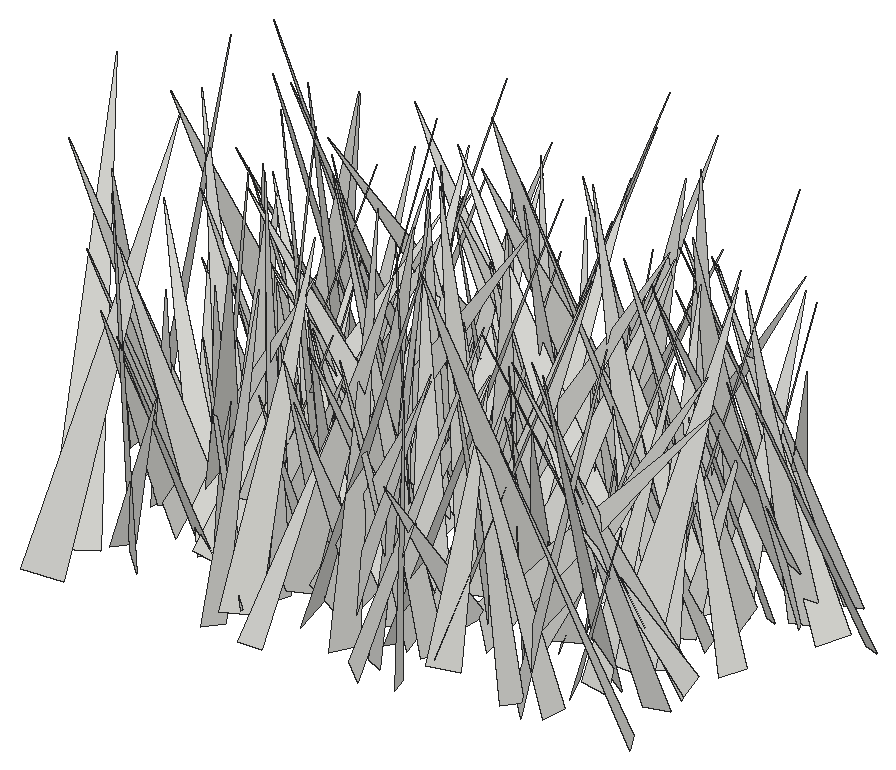
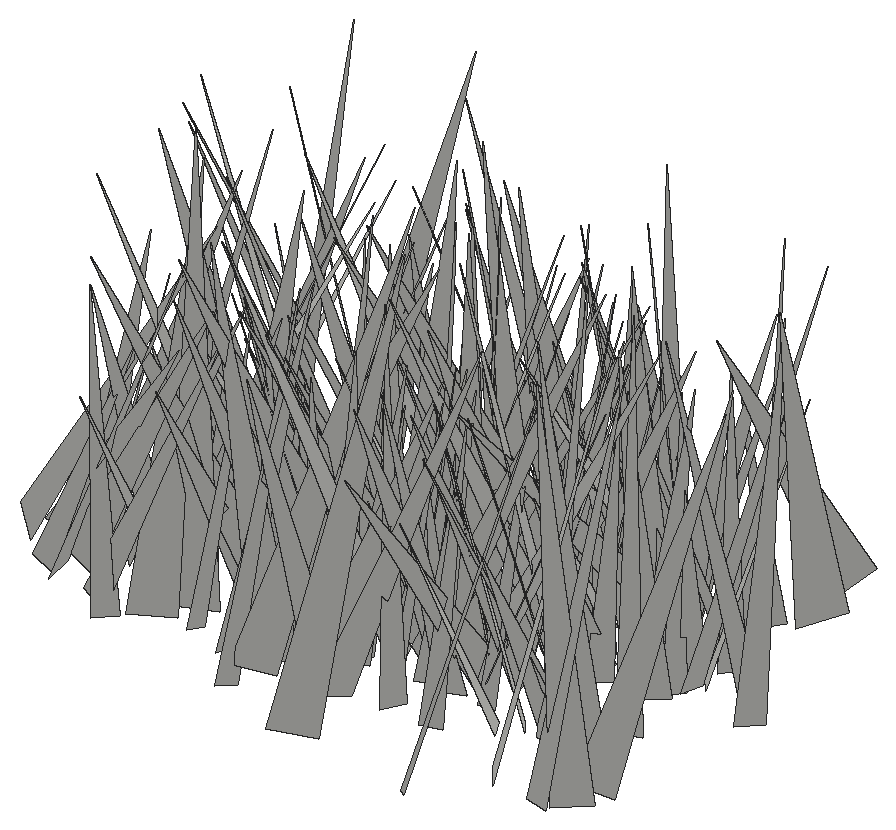
# SketchUp Ruby script. Lengths in inches.
U = 1.inch
M = Sketchup.active_model
def pt(a) = Geom::Point3d.new(a.map { |v| v * U })
def face(e, loops, mat)
  f = e.add_face(loops[0].map { |a| pt(a) })
  loops[1..].each { |l| e.add_face(l.map { |a| pt(a) }).erase! }
  f.material = f.back_material = mat if mat
  f
end
# faces: each face lists its corners as indices into pts; further lists are holes
def faces(e, pts, list, mat = nil) = list.each { |f| face(e, (f[0].is_a?(Array) ? f : [f]).map { |l| l.map { |i| pts[i] } }, mat) }
# xy, xz, yz: faces in a plane at the given z, y or x. An outline is a flat list of corners, or four numbers for a rectangle; further outlines are holes
def ring(l) = l.size == 4 ? [[l[0], l[1]], [l[2], l[1]], [l[2], l[3]], [l[0], l[3]]] : l.each_slice(2).to_a
def flat(e, list, mat, &to3) = list.each { |f| face(e, (f[0].is_a?(Array) ? f : [f]).map { |l| ring(l).map { |u, v| to3.(u, v) } }, mat) }
def xy(e, z, list, mat = nil) = flat(e, list, mat) { |x, y| [x, y, z] }
def xz(e, y, list, mat = nil) = flat(e, list, mat) { |x, z| [x, y, z] }
def yz(e, x, list, mat = nil) = flat(e, list, mat) { |y, z| [x, y, z] }
def lines(e, pts, list) = list.each { |a, b| e.add_line(pt(pts[a]), pt(pts[b])) }
# prism: a flat outline (further loops are holes) pulled along v
def prism(e, loops, v, mat = nil)
  f = face(e, loops, mat); d = Geom::Vector3d.new(v.map { |x| x * U })
  f.pushpull(f.normal.samedirection?(d) ? d.length : -d.length)
end
def box(e, o, s, mat = nil) = prism(e, [[o, [o[0] + s[0], o[1], o[2]], [o[0] + s[0], o[1] + s[1], o[2]], [o[0], o[1] + s[1], o[2]]]], [0, 0, s[2]], mat)
def at(x, y, z, deg = 0) = Geom::Transformation.translation(pt([x, y, z])) * Geom::Transformation.rotation(ORIGIN, Z_AXIS, deg.degrees)
def axes(o, x, y, z) = Geom::Transformation.new([*x, 0, *y, 0, *z, 0, *pt(o).to_a, 1])
def part(name) = M.definitions.add(name)
# library, detail: a bought-in or finely detailed component or shape, given as its bounding box
def library(name, o, s) = part(name).tap { |d| box(d.entities, o, s) }
def detail(e, o, s) = box(e.add_group.entities, o, s)
def put(e, d, t, mat = nil) = e.add_instance(d, t).tap { |i| i.material = mat if mat }
def group(e, t, mat = nil) = e.add_group.tap { |g| g.transformation = t; g.material = mat if mat }.entities
root = M.entities
c1 = part("fur_instance\#9")
p = [[0.8125,0,1.79],[0.67,-0.02,1.48],[0,-0.11,0],[0,0.11,0]]
faces(c1.entities,p,[[0,1,2,3]])
put(root,c1,axes([471.03,125.22,-21.86],[3.80015,2.05854,2.10545],[1.83657,-4.34391,0.93228],[-2.30164,-0.0674,4.22014]))
put(root,c1,axes([459.39,126.23,-21.86],[-4.34525,-4.69158,2.51984],[-5.05188,4.66036,-0.03462],[1.68493,1.87398,6.3946]))
put(root,c1,axes([458.42,126.88,-21.86],[3.1539,-2.32332,0.00557],[-2.32207,-3.15188,0.13648],[0.07647,0.11319,3.91488]))
put(root,c1,axes([479.16,126.97,-21.86],[-4.6266,-2.97065,0.07987],[-2.96143,4.59663,-0.58091],[-0.24706,0.53178,5.46742]))
put(root,c1,axes([465.68,124.31,-21.86],[-2.96386,2.60362,0.59977],[2.15648,2.85999,-1.75873],[1.5774,0.98217,3.53132]))
put(root,c1,axes([463.93,124.63,-21.86],[4.93577,0.48548,2.66433],[-0.37318,-5.36398,1.66873],[-2.68236,1.63958,4.67042]))
put(root,c1,axes([467.54,126.71,-21.66],[3.43659,4.37627,1.35344],[4.55407,-3.08156,-1.59944],[0.49399,-2.03617,5.32951]))
put(root,c1,axes([469.32,125.03,-21.86],[4.12664,4.96749,0.53315],[4.97839,-4.14664,0.10195],[-0.41933,-0.34468,6.45715]))
put(root,c1,axes([466.84,128.88,-21.86],[4.72297,-1.05883,1.70864],[-0.28791,-4.67444,-2.10088],[-1.98939,-1.83725,4.36049]))
put(root,c1,axes([464.3125,125.79,-21.66],[-4.28089,-1.18354,0.47624],[-1.27514,3.91753,-1.72642],[-0.03977,1.79046,4.09221]))
put(root,c1,axes([476.07,129.68,-21.66],[-2.59583,-7.17613,0.91864],[-6.91744,2.74775,1.9178],[2.11891,0.17907,7.38629]))
put(root,c1,axes([460.64,128.33,-21.86],[-1.93771,-4.14246,0.35212],[-4.15628,1.93921,-0.05843],[0.0961,0.34375,4.57288]))
put(root,c1,axes([465.97,127.15,-21.86],[7.81228,1.65656,1.00866],[1.73052,-7.84393,-0.52089],[-0.87571,-0.72239,7.96898]))
put(root,c1,axes([474.79,126.61,-21.86],[4.81614,4.80746,1.57054],[5.00941,-4.83285,-0.56818],[-0.69571,-1.51836,6.78115]))
put(root,c1,axes([469.63,127.7,-21.86],[-4.87581,-1.54153,0.97742],[-1.54685,4.96967,0.12147],[0.96896,0.17664,5.11224]))
put(root,c1,axes([465.83,127.86,-21.66],[0.54416,-5.67013,1.84078],[-5.27926,0.40028,2.79359],[2.76917,1.87733,4.9641]))
put(root,c1,axes([470.54,129.66,-21.66],[3.27584,-2.78093,0.2499],[-2.38988,-2.99185,-1.96583],[-1.44378,-1.35736,3.82103]))
put(root,c1,axes([464.33,125.4375,-21.66],[-4.85985,3.92503,1.53679],[3.59209,5.08366,-1.6245],[2.20555,0.36911,6.032]))
put(root,c1,axes([459.75,130.27,-21.86],[7.63705,-2.12328,0.08153],[-2.0044,-7.29978,-2.35267],[-0.70524,-2.24596,7.56953]))
put(root,c1,axes([468.42,125.72,-21.66],[-7.01527,0.64484,2.20419],[0.06996,7.14138,-1.86657],[2.29551,1.75305,6.79307]))
put(root,c1,axes([476.05,126.86,-21.86],[-6.46685,-0.99912,0.02995],[-0.985,6.33639,-1.3035],[-0.17003,1.29271,6.41243]))
put(root,c1,axes([471.46,126.95,-21.86],[-2.32023,4.26891,1.78267],[4.38145,2.66784,-0.68595],[1.48474,-1.20167,4.81004]))
put(root,c1,axes([457.87,123.47,-21.66],[-6.65412,4.03174,0.74119],[3.28122,6.08544,-3.64454],[2.45722,2.79179,6.87384]))
put(root,c1,axes([464.7,127.56,-21.66],[5.22316,-4.20753,1.34718],[-4.41725,-5.01042,1.47756],[-0.07792,1.998,6.54228]))
put(root,c1,axes([460.52,128.99,-21.66],[-5.0365,1.95588,2.0654],[2.56555,4.93734,1.5806],[1.22852,-2.29236,5.16658]))
put(root,c1,axes([469.27,129.31,-21.86],[-0.62326,-5.57048,0.69706],[-5.46922,0.44429,-1.33972],[-1.26641,0.82277,5.44278]))
put(root,c1,axes([475.54,128.57,-21.86],[4.06757,1.21437,0.51699],[1.31683,-3.847,-1.32426],[-0.08902,-1.4188,4.03313]))
put(root,c1,axes([473.3125,130.72,-21.86],[1.71301,-8.16044,0.92704],[-8.06805,-1.84913,-1.36891],[-1.53583,0.61199,8.22516]))
put(root,c1,axes([458.1,129.83,-21.86],[1.11267,-4.69864,0.20362],[-4.67497,-1.12782,-0.47895],[-0.51316,0.0867,4.80478]))
put(root,c1,axes([461.58,127.625,-21.86],[4.78863,4.89843,2.46119],[5.13986,-5.14824,0.24599],[-1.90629,-1.57608,6.84581]))
put(root,c1,axes([469.78,125.53,-21.66],[4.59054,6.55576,1.84003],[6.00661,-4.94402,2.62946],[-3.20693,0.124,7.5589]))
put(root,c1,axes([464.29,130.58,-21.86],[5.97611,0.87511,2.00016],[1.66713,-5.59279,-2.53411],[-1.40966,-2.90435,5.48252]))
put(root,c1,axes([474.58,126.55,-21.86],[0.67019,6.07953,1.22269],[5.42193,-1.17133,2.85227],[-3.0097,-0.75637,5.41058]))
put(root,c1,axes([464.17,129.51,-21.86],[-0.71572,-3.67555,0.46048],[-3.70429,0.70984,-0.09154],[-0.00255,0.46948,3.74347]))
put(root,c1,axes([478.39,129.18,-21.86],[-1.63613,-6.00923,1.56488],[-6.02721,1.14742,-1.89548],[-1.49415,1.95172,5.93253]))
put(root,c1,axes([464.3,130.44,-21.86],[3.35364,-3.87615,0.32814],[-3.76663,-3.34394,-1.00479],[-0.97195,-0.41544,5.02611]))
put(root,c1,axes([457.41,125.68,-21.86],[-6.50457,4.89284,0.5628],[4.72218,6.46057,-1.59001],[1.39918,0.94188,7.98255]))
put(root,c1,axes([464.77,126.99,-21.66],[-6.75602,-0.97126,1.58692],[-1.43223,6.52998,-2.10085],[1.1876,2.34979,6.49412]))
put(root,c1,axes([464.48,126.44,-21.66],[5.18637,5.57386,2.23152],[5.04396,-5.64447,2.37581],[-3.2567,0.13438,7.23339]))
put(root,c1,axes([457.59,130.06,-21.86],[4.72712,-1.54603,0.79765],[-1.39638,-4.74943,-0.93014],[-1.03759,-0.65178,4.88576]))
put(root,c1,axes([470.87,127.18,-21.66],[-7.866,-1.33504,0.19154],[-1.32695,7.45779,-2.51268],[-0.24134,2.50839,7.5725]))
put(root,c1,axes([458.58,129.0625,-21.86],[3.98085,5.13777,1.04709],[4.9615,-3.26572,-2.83883],[1.69606,-2.50573,5.84679]))
put(root,c1,axes([462.55,129.47,-21.86],[2.89103,-3.61881,0.35286],[-3.55779,-2.72252,1.22815],[0.74997,1.03461,4.46604]))
put(root,c1,axes([478.27,130.91,-21.86],[-6.15592,-2.89241,0.11132],[-2.84807,6.09927,0.98037],[0.51666,-0.84058,6.73054]))
put(root,c1,axes([460.89,127.93,-21.86],[-0.53064,3.51066,0.60828],[3.36851,0.69471,-1.0709],[1.16098,-0.41106,3.38519]))
put(root,c1,axes([470.97,129.54,-21.66],[5.03462,6.0848,0.40692],[5.07887,-3.8915,-4.64748],[3.37572,-3.22012,6.38538]))
put(root,c1,axes([478.5625,130.72,-21.66],[-4.09373,-0.36711,0.23804],[-0.24891,3.79616,1.57392],[0.35983,-1.55061,3.79686]))
put(root,c1,axes([470.94,130.18,-21.86],[-4.44854,-2.43941,1.67916],[-2.34276,4.75236,0.69742],[1.81157,0.15557,5.02532]))
put(root,c1,axes([460.875,129.9,-21.86],[3.92094,-4.8226,1.73149],[-5.06492,-3.97791,0.39007],[-0.77596,1.59628,6.20315]))
put(root,c1,axes([473.91,128.03,-21.86],[-4.19914,-2.372,1.71601],[-2.90919,3.71707,-1.98087],[0.32817,2.60017,4.39719]))
put(root,c1,axes([461.1875,128.28,-21.86],[-3.00084,5.06154,0.45444],[5.0055,2.85272,1.2797],[-0.87785,-1.03611,5.74339]))
put(root,c1,axes([457.86,131.78,-21.86],[-7.05336,-2.15617,1.71578],[-1.62887,7.06566,2.18314],[2.22256,-1.66441,7.04506]))
put(root,c1,axes([470.6,127.92,-21.86],[6.55777,3.05775,0.67545],[3.00333,-6.58518,0.65252],[-0.88663,0.30968,7.20614]))
put(root,c1,axes([467,129.73,-21.86],[2.81827,1.89164,1.24112],[2.11841,-2.90244,-0.38665],[-0.79437,-1.02901,3.37216]))
put(root,c1,axes([457.72,131.27,-21.86],[-3.97352,-3.33663,0.47318],[-3.25036,3.98768,0.8243],[0.89005,-0.33346,5.12275]))
put(root,c1,axes([467.76,130.1,-21.86],[4.83002,3.67653,3.08875],[4.26917,-5.29337,-0.3752],[-2.19806,-2.20219,6.05848]))
put(root,c1,axes([468.93,129.48,-21.86],[3.45962,-4.50001,2.91683],[-5.02174,-3.93643,-0.1168],[-1.88153,2.2319,5.67498]))
put(root,c1,axes([469.73,128.25,-21.86],[2.30646,3.84948,0.31393],[3.83736,-2.32546,0.32205],[-0.43787,-0.10267,4.47599]))
put(root,c1,axes([468.7,127.95,-21.66],[-4.6642,0.46344,0.8289],[0.1067,4.38406,-1.85075],[0.94364,1.79496,4.30631]))
put(root,c1,axes([464.67,131.57,-21.66],[0.15208,-7.64456,1.76209],[-7.47072,0.39677,2.36609],[2.3943,1.72356,7.27077]))
put(root,c1,axes([472.29,130.5,-21.86],[3.77376,6.10396,1.49671],[5.76595,-2.66802,-3.65722],[2.50047,-3.05991,6.17449]))
put(root,c1,axes([464.375,129.37,-21.86],[-0.0394,4.36961,1.02441],[4.32756,-0.23455,1.1669],[-1.18959,-0.99797,4.2111]))
put(root,c1,axes([462.5,131.08,-21.86],[2.53184,-2.74895,1.13947],[-2.76231,-2.72751,-0.44237],[-1.1067,0.51894,3.71097]))
put(root,c1,axes([461.92,131.78,-21.86],[-4.44345,-1.97155,1.25823],[-1.71315,4.58269,1.13072],[1.59225,-0.57131,4.72787]))
put(root,c1,axes([469.61,128.93,-21.66],[-7.1733,-2.93015,0.73361],[-2.97558,6.52972,-3.01478],[-0.51951,3.05896,7.13815]))
put(root,c1,axes([465.625,128.45,-21.86],[-7.24108,-2.76695,1.69952],[-3.23599,6.49389,-3.21487],[0.2698,3.62643,7.05364]))
put(root,c1,axes([470.57,133.06,-21.66],[5.43533,-0.93824,0.08866],[-0.80913,-4.91198,-2.3767],[-0.48317,-2.32876,4.97739]))
put(root,c1,axes([454.73,132.75,-21.66],[6.40589,-1.32849,1.4611],[-0.83624,-6.31798,-2.07823],[-1.78897,-1.80373,6.20333]))
put(root,c1,axes([476.03,128.99,-21.86],[1.01663,5.56132,0.68679],[5.60282,-1.02017,-0.03274],[-0.09106,-0.68151,5.65338]))
put(root,c1,axes([460.71,131.17,-21.86],[4.5818,0.64032,0.1617],[0.65902,-4.5067,-0.82732],[-0.04299,-0.84188,4.55176]))
put(root,c1,axes([463.44,130.95,-21.66],[-0.2537,5.53184,2.90433],[5.7111,-0.97344,2.35297],[-2.53371,-2.74807,5.0129]))
put(root,c1,axes([469.34,126.875,-21.66],[6.78257,3.66457,1.14232],[2.83952,-6.35069,3.51329],[-2.58286,2.6414,6.86216]))
put(root,c1,axes([458.11,132.36,-21.86],[4.73789,-1.18845,0.72275],[-0.9672,-4.65874,-1.32025],[-0.99966,-1.12521,4.70287]))
put(root,c1,axes([469.47,131.43,-21.86],[-2.10134,6.53759,3.4605],[7.38552,2.05442,0.60354],[0.41142,-3.48856,6.84043]))
put(root,c1,axes([473.1,131.03,-21.86],[7.00496,3.81978,0.96353],[3.93839,-6.83549,-1.53416],[-0.09034,-1.80938,7.82984]))
put(root,c1,axes([465.2,129.82,-21.86],[-5.62336,3.63446,0.06059],[3.63174,5.6129,0.37548],[-0.15301,-0.3482,6.6851]))
put(root,c1,axes([462.27,127.52,-21.66],[5.32818,4.49942,0.50618],[3.89144,-4.95023,3.04014],[-2.31467,2.03493,6.2763]))
put(root,c1,axes([470.91,133.2,-21.86],[0.77798,-4.23548,0.16889],[-4.23878,-0.77834,0.00619],[-0.02442,0.16723,4.30633]))
put(root,c1,axes([476.41,131.09,-21.86],[-3.97928,1.73175,0.54979],[1.73454,4.01483,-0.09183],[0.54094,-0.13447,4.3388]))
put(root,c1,axes([476.41,130.29,-21.66],[-2.09917,6.50868,2.06271],[6.47308,2.58358,-1.56477],[2.17184,-1.40938,6.65739]))
put(root,c1,axes([465.58,131.63,-21.86],[3.09859,-2.8989,0.71648],[-2.92503,-2.73871,1.56906],[0.60101,1.61681,3.94246]))
put(root,c1,axes([462.38,131.14,-21.86],[5.69226,-5.26322,0.96159],[-5.00885,-4.7486,3.65927],[1.88086,3.28288,6.8347]))
put(root,c1,axes([463.44,132.83,-21.86],[-5.49942,-3.45806,0.94275],[-3.51329,5.5426,-0.16378],[0.70973,0.64178,6.49422]))
put(root,c1,axes([466.11,133.66,-21.86],[-7.08449,-0.21202,0.14595],[-0.16992,6.87165,1.73429],[0.19334,-1.72965,6.8722]))
put(root,c1,axes([458.72,130.62,-21.86],[-4.24883,1.88722,0.42776],[1.75815,4.19597,-1.04876],[0.80838,0.79335,4.52927]))
put(root,c1,axes([472.27,134.57,-21.86],[-3.47678,-4.99975,0.07246],[-4.93171,3.44331,0.95532],[0.82523,-0.48669,6.01439]))
put(root,c1,axes([471.5,132.2,-21.86],[1.72384,-3.5656,0.8716],[-3.29525,-1.07913,2.10276],[1.61693,1.60212,3.35612]))
put(root,c1,axes([463.73,133.1,-21.86],[0.72019,-3.80208,0.86926],[-3.795,-0.88705,-0.73566],[-0.89965,0.69817,3.79912]))
put(root,c1,axes([460.47,133.25,-21.86],[3.6116,-2.54944,1.03868],[-2.46348,-3.75778,-0.65768],[-1.22872,0.0404,4.37159]))
put(root,c1,axes([460.22,130.63,-21.86],[-6.64184,2.29308,0.28161],[2.23011,6.58737,-1.04152],[0.60342,0.8944,6.94892]))
put(root,c1,axes([468.97,132.04,-21.66],[2.35297,-5.60644,2.50548],[-6.03434,-1.6135,2.05656],[1.13856,3.03489,5.72182]))
put(root,c1,axes([458.47,133.07,-21.86],[2.75053,-5.09352,1.52718],[-5.31748,-2.64324,0.76119],[-0.02665,1.70616,5.73847]))
put(root,c1,axes([478.82,132.51,-21.86],[-3.90024,1.94852,0.94584],[2.05782,3.9414,0.36592],[0.67579,-0.75618,4.3445]))
put(root,c1,axes([460.8,128.95,-21.86],[-3.50989,5.55769,0.51718],[4.45011,3.15505,-3.70364],[3.36927,1.62248,5.4305]))
put(root,c1,axes([456.37,130.81,-21.66],[6.51752,3.06728,2.32468],[2.5593,-6.86862,1.88745],[-2.87443,0.8392,6.95153]))
put(root,c1,axes([465.4,133.67,-21.86],[4.72126,-4.87179,1.88096],[-5.03873,-4.91595,-0.08523],[-1.37242,1.28908,6.78361]))
put(root,c1,axes([467.125,133.32,-21.86],[4.55418,4.59674,3.34406],[5.23121,-5.06575,-0.16086],[-2.22422,-2.50228,6.46875]))
put(root,c1,axes([466.09,129.48,-21.66],[-5.16112,5.15909,0.10388],[4.87926,4.92701,-2.27629],[1.67923,1.54029,6.93338]))
put(root,c1,axes([463.09,135.64,-21.66],[-4.74866,-3.13825,0.27488],[-2.86364,4.50737,1.98925],[1.31291,-1.51952,5.33303]))
put(root,c1,axes([476.84,131.19,-21.86],[-5.4201,3.31702,1.28358],[3.06796,5.54385,-1.37151],[1.7994,0.53923,6.20476]))
put(root,c1,axes([461.71,130.85,-21.86],[3.36886,3.17868,0.5186],[2.75759,-3.23451,1.91201],[-1.66392,1.0752,4.2187]))
put(root,c1,axes([477.375,133.13,-21.66],[-7.14593,-4.06809,0.00282],[-3.91681,6.87864,-2.22635],[-1.09909,1.93614,7.91562]))
put(root,c1,axes([477.14,135.26,-21.86],[-7.14717,-1.7401,1.8273],[-1.33254,7.26397,1.70532],[2.14274,-1.28679,7.15555]))
put(root,c1,axes([457.36,135.61,-21.66],[-1.15928,-6.64992,1.1524],[-6.36185,1.46707,2.06591],[2.25307,0.72087,6.42631]))
put(root,c1,axes([467.94,134.37,-21.86],[0.59547,-6.22896,1.95156],[-6.50827,-0.41619,0.65745],[0.50087,1.99748,6.22272]))
put(root,c1,axes([458.6,134.49,-21.86],[-0.08918,-3.86635,0.81214],[-3.84672,-0.10019,-0.89937],[-0.90053,0.81086,3.76135]))
put(root,c1,axes([468.73,131.03,-21.86],[3.68113,4.53912,0.36663],[4.24955,-3.59341,1.82137],[-1.63686,0.87892,5.5531]))
put(root,c1,axes([470.48,132.08,-21.86],[1.11802,6.55656,0.88639],[6.4324,-0.86675,-1.70208],[1.54866,-1.13332,6.42972]))
put(root,c1,axes([473.61,131.5,-21.86],[4.34106,2.99141,0.28027],[2.79242,-4.19877,1.56351],[-1.10882,1.13738,5.03476]))
put(root,c1,axes([474.71,133.61,-21.66],[-1.73257,6.85044,2.42635],[7.20837,1.30251,1.46979],[-0.92468,-2.68187,6.91158]))
put(root,c1,axes([467.07,134.43,-21.86],[4.40787,6.56573,1.54887],[6.23945,-3.26461,-3.91775],[2.5646,-3.34225,6.86945]))
put(root,c1,axes([463.53,135.89,-21.86],[-3.69679,-5.87263,0.02895],[-5.78236,3.6339,-1.23044],[-1.02613,0.67962,6.82936]))
put(root,c1,axes([476.2,133.29,-21.86],[3.26385,-1.40609,1.47007],[-1.85279,-3.20219,1.05074],[-0.83985,1.59994,3.39496]))
put(root,c1,axes([475.11,133.7,-21.86],[4.24313,0.45781,1.20359],[0.34307,-4.39664,0.46288],[-1.24117,0.34981,4.24258]))
put(root,c1,axes([473.4,131.81,-21.86],[4.43621,4.25023,1.48293],[3.65379,-4.61591,2.29927],[-2.62932,0.75659,5.69717]))
put(root,c1,axes([464.72,135.63,-21.66],[-1.05562,-3.90874,0.84941],[-3.49411,1.32871,1.77194],[1.94702,0.26528,3.64044]))
put(root,c1,axes([461.46,133.84,-21.86],[6.44327,3.68852,1.42181],[3.82977,-6.4983,-0.49739],[-0.97955,-1.14429,7.40767]))
put(root,c1,axes([468.34,132.28,-21.86],[-6.09623,-2.24198,1.5344],[-2.70516,5.35755,-2.91953],[0.25098,3.28863,5.80232]))
put(root,c1,axes([473.16,133.97,-21.66],[-5.71693,5.39586,0.3581],[5.20349,5.34707,2.50186],[-1.47216,-2.05434,7.45247]))
put(root,c1,axes([460.95,132.52,-21.86],[-2.94733,3.27814,0.42411],[3.06608,2.92358,-1.29021],[1.23501,0.56503,4.21525]))
put(root,c1,axes([471.34,133.88,-21.86],[-0.34348,3.88251,1.09091],[4.02925,0.37671,-0.07204],[0.17064,-1.07988,3.89701]))
put(root,c1,axes([466.83,135.05,-21.86],[2.18952,-4.24382,2.13551],[-4.35668,-2.73133,-0.96101],[-1.89466,1.3763,4.67766]))
put(root,c1,axes([478.28,137.07,-21.86],[-1.07248,-7.00957,0.36815],[-6.96342,1.01561,-0.94825],[-0.88342,0.50425,7.02746]))
put(root,c1,axes([462.24,136.78,-21.86],[-1.799,-4.93024,0.4482],[-4.7112,1.85147,1.45641],[1.52075,-0.09654,5.04207]))
put(root,c1,axes([465.61,135.81,-21.86],[-3.74944,-6.99723,1.04952],[-6.92154,3.38084,-2.18706],[-1.468,1.93125,7.63127]))
put(root,c1,axes([475.8,134.91,-21.86],[-3.5373,3.73043,1.14853],[3.88761,3.22863,1.48666],[-0.34887,-1.84596,4.92122]))
put(root,c1,axes([474.16,136.36,-21.86],[3.81403,-1.87609,0.65313],[-1.66249,-3.78837,-1.17367],[-1.0874,-0.78844,4.08523]))
put(root,c1,axes([463.67,131.76,-21.86],[6.96857,3.90701,1.2479],[3.36407,-6.85211,2.66731],[-2.34628,1.77954,7.53068]))
put(root,c1,axes([468.68,136.93,-21.86],[6.75782,0.35235,2.65885],[1.16075,-6.88187,-2.03823],[-2.41791,-2.31896,6.45275]))
put(root,c1,axes([472.32,135.14,-21.86],[3.33409,-2.8819,1.80128],[-3.12207,-3.59416,0.02846],[-1.34262,1.20116,4.40689]))
put(root,c1,axes([464.61,136.71,-21.86],[2.27929,-4.31761,0.37807],[-4.29346,-2.30768,-0.46977],[-0.59235,0.11282,4.85966]))
put(root,c1,axes([471.8,135.89,-21.86],[-0.47471,-3.8388,0.84095],[-3.92781,0.49062,0.02236],[0.12592,0.83177,3.86797]))
put(root,c1,axes([464.46,133.6,-21.66],[3.7445,3.22853,1.26331],[2.91821,-3.9391,1.41711],[-1.87174,0.31742,4.73672]))
put(root,c1,axes([475.45,132.63,-21.86],[6.6915,4.26773,1.20587],[3.94044,-6.72308,1.92792],[-2.03484,1.01512,7.69888]))
put(root,c1,axes([468.5625,132.58,-21.66],[5.48783,2.36239,1.1528],[1.72376,-5.24883,2.55038],[-1.98455,1.97355,5.40302]))
put(root,c1,axes([478.37,136.65,-21.86],[-4.22717,-2.44585,1.01456],[-2.28976,4.33627,0.91336],[1.32985,-0.3083,4.79759]))
put(root,c1,axes([459.29,137.42,-21.86],[-3.46246,-6.72611,1.90114],[-6.59046,3.84836,1.61233],[2.32826,0.89059,7.39118]))
put(root,c1,axes([467.36,136.71,-21.86],[3.88583,-1.17381,1.38743],[-0.79486,-4.04284,-1.19419],[-1.63432,-0.82466,3.87962]))
put(root,c1,axes([464.13,136.43,-21.86],[1.922,-3.18961,0.22781],[-3.1707,-1.86642,0.61867],[0.41494,0.51232,3.67219]))
put(root,c1,axes([460.9,134.78,-21.86],[3.76051,3.97563,0.83952],[4.01253,-3.81366,0.08642],[-0.64034,-0.54974,5.47171]))
put(root,c1,axes([481.32,136.47,-21.86],[-4.75874,-5.64309,0.42264],[-5.39038,4.3522,-2.58279],[-1.72245,1.97043,6.91515]))
put(root,c1,axes([477.63,135.95,-21.86],[-3.98273,-4.40716,0.90523],[-4.3967,3.55588,-2.0321],[-0.95477,2.0093,5.58174]))
put(root,c1,axes([467.36,137.21,-21.86],[3.57581,-3.48366,1.446],[-3.33217,-3.85124,-1.03819],[-1.76733,0.21279,4.88308]))
put(root,c1,axes([478.72,136.43,-21.86],[0.19192,-5.71021,2.24229],[-6.02696,-0.59408,-0.99702],[-1.14462,2.17066,5.62577]))
put(root,c1,axes([463.16,135.22,-21.86],[3.02903,2.92229,1.12241],[2.89072,-3.2105,0.55771],[-1.2014,-0.35704,4.17178]))
put(root,c1,axes([468.7,135.99,-21.86],[4.45392,4.12687,0.87812],[4.21021,-4.26347,-1.31776],[0.27618,-1.55927,5.92722]))
put(root,c1,axes([469.38,139.8,-21.66],[6.1806,-4.85252,1.92283],[-3.89661,-6.27237,-3.30423],[-3.47285,-1.59827,7.12944]))
put(root,c1,axes([473.58,137.56,-21.86],[2.47243,-7.62212,2.09201],[-7.90302,-2.41845,0.52868],[-0.12434,2.1542,7.99563]))
put(root,c1,axes([468.61,133.97,-21.66],[-3.2571,5.60614,0.8435],[5.30317,3.35677,-1.83235],[2.00417,0.22864,6.21933]))
put(root,c1,axes([457.75,137.04,-21.86],[-0.42435,-6.57592,2.54627],[-6.78158,1.0798,1.65847],[1.93298,2.34469,6.37748]))
put(root,c1,axes([474.3,138.8,-21.86],[5.27875,-5.42072,0.96709],[-5.29735,-5.36505,-1.15714],[-1.50251,-0.12916,7.47733]))
put(root,c1,axes([469.56,134.87,-21.86],[0.02975,6.47261,1.15989],[6.34372,-0.33363,1.69906],[-1.73125,-1.11127,6.2457]))
put(root,c1,axes([470.91,133.17,-21.86],[7.42059,-0.17453,3.00871],[-1.57677,-7.03899,3.48057],[-2.56838,3.81708,6.55601]))
put(root,c1,axes([462.03,135.04,-21.66],[5.46763,0.70402,1.09334],[0.38726,-5.3924,1.5356],[-1.2414,1.41859,5.29457]))
put(root,c1,axes([455.94,139.21,-21.66],[2.22572,-6.24997,0.53761],[-6.03536,-2.28904,-1.62473],[-1.71046,-0.05581,6.43243]))
put(root,c1,axes([470.31,135.22,-21.86],[-5.05186,2.37101,0.85511],[2.22237,5.09377,-0.9944],[1.18912,0.55319,5.49128]))
put(root,c1,axes([472.49,138.8125,-21.66],[5.01646,-0.03484,2.02413],[0.79085,-4.94522,-2.0451],[-1.86357,-2.19241,4.58078]))
put(root,c1,axes([465.53,137.28,-21.86],[-2.97615,-4.05495,1.48787],[-4.26463,3.04523,-0.23114],[0.68511,1.34083,5.02461]))
put(root,c1,axes([467.9,133.56,-21.66],[7.02675,2.35333,1.41841],[1.60681,-6.67867,3.12071],[-2.22895,2.60433,6.72121]))
put(root,c1,axes([471.3,135.86,-21.86],[6.564,-1.73993,0.0582],[-1.67851,-6.26496,2.01239],[0.46191,1.95953,6.48565]))
put(root,c1,axes([460.51,137.01,-21.86],[4.49917,3.28934,0.87918],[3.40387,-4.3112,-1.28935],[0.07989,-1.55853,5.42216]))
put(root,c1,axes([476.34,135.57,-21.86],[-1.65909,5.33475,1.21269],[5.33342,1.85943,-0.88312],[1.21852,-0.87506,5.51654]))
put(root,c1,axes([462.85,138.875,-21.86],[-0.56005,-4.94681,0.27227],[-4.82604,0.60667,1.09544],[1.12,0.14049,4.85639]))
put(root,c1,axes([463.66,136.76,-21.86],[0.44835,5.06558,1.88586],[5.29017,-0.02286,-1.19629],[1.10933,-1.93829,4.94267]))
put(root,c1,axes([465.25,134.99,-21.86],[-2.73527,5.15415,0.70761],[4.98067,2.82527,-1.3261],[1.50298,0.0175,5.68229]))
put(root,c1,axes([464.4,138.86,-21.66],[6.47505,-0.26988,1.20187],[0.07267,-6.33614,-1.81428],[-1.22965,-1.79557,6.22153]))
put(root,c1,axes([480,136.1875,-21.86],[-2.08516,6.03207,0.25096],[5.29839,1.7011,3.1353],[-2.89412,-1.23172,5.5591]))
put(root,c1,axes([478.52,138.3,-21.86],[-6.23663,-1.3966,0.55844],[-1.37103,6.25805,0.33911],[0.61857,-0.21031,6.38209]))
put(root,c1,axes([468.99,137.09,-21.86],[6.19791,-1.23637,0.25272],[-1.26158,-6.10069,1.0939],[-0.02993,1.12232,6.22464]))
put(root,c1,axes([467.48,139.22,-21.86],[1.50286,-5.49819,1.33251],[-5.18917,-1.88889,-1.94134],[-2.25347,0.68284,5.35909]))
put(root,c1,axes([473.23,135.01,-21.86],[-4.89219,1.92037,1.37183],[1.09822,4.64707,-2.5888],[2.08893,2.05431,4.57377]))
put(root,c1,axes([479.16,138.3,-21.86],[-0.99125,-4.30354,0.98962],[-4.28593,0.69339,-1.27766],[-1.06332,1.21702,4.22737]))
put(root,c1,axes([478.18,137.7,-21.66],[-1.48445,-5.73193,2.26963],[-5.6541,0.33538,-2.85107],[-2.45713,2.69116,5.18942]))
put(root,c1,axes([471.02,138.85,-21.86],[-6.42976,0.15301,2.02637],[0.5172,6.6259,1.14077],[1.96522,-1.24316,6.3296]))
put(root,c1,axes([459.3,140.14,-21.86],[-6.10704,-5.17922,1.29191],[-4.99805,6.23748,1.37932],[1.87424,-0.24245,7.88782]))
put(root,c1,axes([458.38,137.05,-21.86],[3.26284,4.45559,0.15103],[4.26787,-3.06768,-1.7017],[1.28856,-1.1217,5.25381]))
put(root,c1,axes([466.125,136.19,-21.86],[7.5502,3.19495,0.69372],[3.12341,-7.56468,0.84526],[-0.96605,0.51231,8.15468]))
put(root,c1,axes([475.43,139.75,-21.86],[5.22724,-1.35677,0.09683],[-1.28473,-5.05093,-1.4184],[-0.44684,-1.34966,5.21086]))
put(root,c1,axes([466.6,139.25,-21.86],[-6.62778,2.24684,1.33683],[2.5489,6.36376,1.94128],[0.58185,-2.2841,6.72363]))
put(root,c1,axes([469.34,138.625,-21.86],[2.95876,-6.29379,1.88961],[-6.54545,-2.63888,1.45948],[0.58268,2.31543,6.79971]))
put(root,c1,axes([469.64,140.81,-21.86],[6.21031,-0.46369,2.15458],[0.49806,-5.98034,-2.72263],[-2.14689,-2.7287,5.60092]))
put(root,c1,axes([476.41,139.13,-21.86],[-1.75901,-5.06572,0.78099],[-4.97011,1.48393,-1.5689],[-1.25276,1.22556,5.12778]))
put(root,c1,axes([460.67,143.05,-21.66],[-6.33754,-5.19611,0.8236],[-4.02771,5.62162,4.47406],[3.3846,-3.03975,6.86635]))
put(root,c1,axes([456.85,141,-21.66],[-3.15588,-6.30761,0.73503],[-6.08642,3.23856,1.65924],[1.81157,-0.10755,6.85511]))
put(root,c1,axes([461.11,137.67,-21.86],[3.47844,1.93474,0.04271],[1.93521,-3.47755,-0.07868],[0.00093,-0.08952,3.97952]))
put(root,c1,axes([467.08,138.92,-21.66],[3.19208,-3.97574,0.46961],[-3.91795,-2.97897,1.41133],[0.82265,1.2392,4.89939]))
put(root,c1,axes([463.33,135.24,-21.86],[-5.44791,2.04028,1.98238],[0.64646,5.0587,-3.42987],[2.77031,2.83181,4.69878]))
put(root,c1,axes([460.09,136.16,-21.86],[-4.70225,1.57903,0.9136],[0.9953,4.33742,-2.37389],[1.52885,2.03289,4.35536]))
put(root,c1,axes([455.875,140.38,-21.66],[2.61473,-6.42495,0.46001],[-6.33227,-2.47287,1.45453],[1.18065,0.96609,6.78241]))
put(root,c1,axes([476.03,136.25,-21.66],[3.78632,3.0497,0.88341],[2.42458,-3.66486,2.25998],[-2.05,1.29824,4.30457]))
put(root,c1,axes([466.01,141.98,-21.86],[5.79186,-5.56058,1.06137],[-5.14067,-5.80215,-2.34538],[-2.37068,-1.00358,7.67886]))
